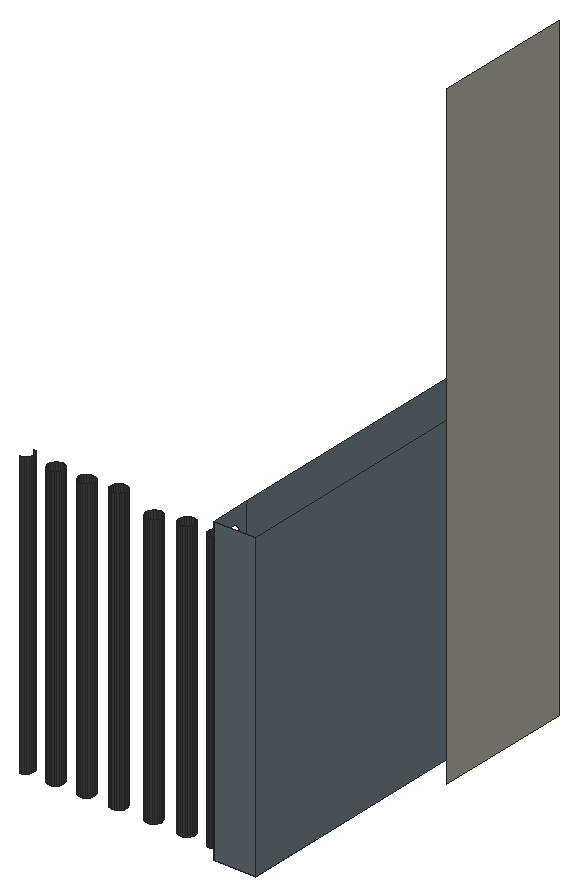
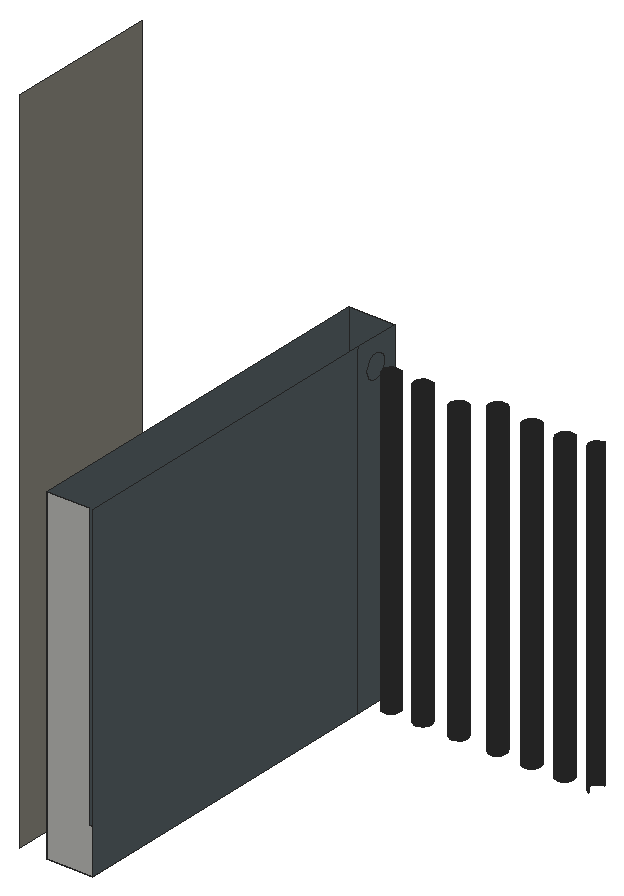
# SketchUp Ruby script. Lengths in inches.
U = 1.inch
M = Sketchup.active_model
def pt(a) = Geom::Point3d.new(a.map { |v| v * U })
def face(e, loops, mat)
  f = e.add_face(loops[0].map { |a| pt(a) })
  loops[1..].each { |l| e.add_face(l.map { |a| pt(a) }).erase! }
  f.material = f.back_material = mat if mat
  f
end
# faces: each face lists its corners as indices into pts; further lists are holes
def faces(e, pts, list, mat = nil) = list.each { |f| face(e, (f[0].is_a?(Array) ? f : [f]).map { |l| l.map { |i| pts[i] } }, mat) }
# xy, xz, yz: faces in a plane at the given z, y or x. An outline is a flat list of corners, or four numbers for a rectangle; further outlines are holes
def ring(l) = l.size == 4 ? [[l[0], l[1]], [l[2], l[1]], [l[2], l[3]], [l[0], l[3]]] : l.each_slice(2).to_a
def flat(e, list, mat, &to3) = list.each { |f| face(e, (f[0].is_a?(Array) ? f : [f]).map { |l| ring(l).map { |u, v| to3.(u, v) } }, mat) }
def xy(e, z, list, mat = nil) = flat(e, list, mat) { |x, y| [x, y, z] }
def xz(e, y, list, mat = nil) = flat(e, list, mat) { |x, z| [x, y, z] }
def yz(e, x, list, mat = nil) = flat(e, list, mat) { |y, z| [x, y, z] }
def lines(e, pts, list) = list.each { |a, b| e.add_line(pt(pts[a]), pt(pts[b])) }
# prism: a flat outline (further loops are holes) pulled along v
def prism(e, loops, v, mat = nil)
  f = face(e, loops, mat); d = Geom::Vector3d.new(v.map { |x| x * U })
  f.pushpull(f.normal.samedirection?(d) ? d.length : -d.length)
end
def box(e, o, s, mat = nil) = prism(e, [[o, [o[0] + s[0], o[1], o[2]], [o[0] + s[0], o[1] + s[1], o[2]], [o[0], o[1] + s[1], o[2]]]], [0, 0, s[2]], mat)
def at(x, y, z, deg = 0) = Geom::Transformation.translation(pt([x, y, z])) * Geom::Transformation.rotation(ORIGIN, Z_AXIS, deg.degrees)
def axes(o, x, y, z) = Geom::Transformation.new([*x, 0, *y, 0, *z, 0, *pt(o).to_a, 1])
def part(name) = M.definitions.add(name)
# library, detail: a bought-in or finely detailed component or shape, given as its bounding box
def library(name, o, s) = part(name).tap { |d| box(d.entities, o, s) }
def detail(e, o, s) = box(e.add_group.entities, o, s)
def put(e, d, t, mat = nil) = e.add_instance(d, t).tap { |i| i.material = mat if mat }
def group(e, t, mat = nil) = e.add_group.tap { |g| g.transformation = t; g.material = mat if mat }.entities
root = M.entities
M.materials.add("[Color M07]").color = [58, 58, 58]
M.materials.add("[Formica Graystone]").color = [149, 146, 135]
M.materials.add("[Formica Speckled Grey]").color = [94, 105, 111]
xy(root,557.29,[[289.43,116.47,292.74,144.04],[275.6,117.55,275.4375,117.57,275.29,117.63,275.16,117.73,275.06,117.86,275,118.01,274.98,118.17,275,118.33,275.06,118.48,275.16,118.61,275.29,118.71,275.4375,118.77,275.6,118.8,275.76,118.77,275.91,118.71,276.04,118.61,276.14,118.48,276.2,118.33,276.23,118.17,276.2,118.01,276.14,117.86,276.04,117.73,275.91,117.63,275.76,117.57],[278.04,117.55,277.875,117.57,277.73,117.63,277.6,117.73,277.5,117.86,277.43,118.01,277.41,118.17,277.43,118.33,277.5,118.48,277.6,118.61,277.73,118.71,277.875,118.77,278.04,118.8,278.2,118.77,278.35,118.71,278.48,118.61,278.58,118.48,278.64,118.33,278.66,118.17,278.64,118.01,278.58,117.86,278.48,117.73,278.35,117.63,278.2,117.57],[280.54,117.55,280.375,117.57,280.23,117.63,280.1,117.73,280,117.86,279.93,118.01,279.91,118.17,279.93,118.33,280,118.48,280.1,118.61,280.23,118.71,280.375,118.77,280.54,118.8,280.7,118.77,280.85,118.71,280.98,118.61,281.08,118.48,281.14,118.33,281.16,118.17,281.14,118.01,281.08,117.86,280.98,117.73,280.85,117.63,280.7,117.57],[283.35,117.55,283.1875,117.57,283.04,117.63,282.91,117.73,282.81,117.86,282.75,118.01,282.73,118.17,282.75,118.33,282.81,118.48,282.91,118.61,283.04,118.71,283.1875,118.77,283.35,118.8,283.51,118.77,283.66,118.71,283.79,118.61,283.89,118.48,283.95,118.33,283.98,118.17,283.95,118.01,283.89,117.86,283.79,117.73,283.66,117.63,283.51,117.57],
  [285.98,117.55,285.8125,117.57,285.66,117.63,285.53,117.73,285.43,117.86,285.37,118.01,285.35,118.17,285.37,118.33,285.43,118.48,285.53,118.61,285.66,118.71,285.8125,118.77,285.98,118.8,286.14,118.77,286.29,118.71,286.42,118.61,286.52,118.48,286.58,118.33,286.6,118.17,286.58,118.01,286.52,117.86,286.42,117.73,286.29,117.63,286.14,117.57],[288.29,117.55,288.125,117.57,287.98,117.63,287.85,117.73,287.75,117.86,287.68,118.01,287.66,118.17,287.68,118.33,287.75,118.48,287.85,118.61,287.98,118.71,288.125,118.77,288.29,118.8,288.45,118.77,288.6,118.71,288.73,118.61,288.83,118.48,288.89,118.33,288.91,118.17,288.89,118.01,288.83,117.86,288.73,117.73,288.6,117.63,288.45,117.57]])
xz(root,116.47,[[289.43,557.29,292.74,581.29]],"[Formica Speckled Grey]")
xz(root,144.04,[[289.43,557.29,292.74,557.29,292.74,581.29,289.71,581.29,289.71,560.54,289.43,560.54]])
yz(root,289.43,[[[116.47,557.29,119.78,581.29],[118.19,578.44,118.41,578.47,118.62,578.56,118.8,578.7,118.94,578.88,119.03,579.09,119.06,579.32,119.03,579.54,118.94,579.76,118.8,579.9375,118.62,580.08,118.41,580.16,118.19,580.19,117.96,580.16,117.75,580.08,117.57,579.9375,117.43,579.76,117.34,579.54,117.31,579.32,117.34,579.09,117.43,578.88,117.57,578.7,117.75,578.56,117.96,578.47]],[119.78,557.29,144.04,581.29]],"[Formica Speckled Grey]")
yz(root,292.74,[[116.47,557.29,144.04,581.29]],"[Formica Speckled Grey]")
yz(root,294.7,[[132.97,557.29,144.04,606.58]],"[Formica Graystone]")
p = [[273.23,117.55,557.29],[273.39,117.57,557.29],[273.39,117.57,578.7],[273.39,117.57,579.76],[273.23,117.55,579.76],[275.4375,117.57,557.29],
  [275.6,117.55,557.29],[275.6,117.55,579.54],[275.4375,117.57,579.54],[275.4375,117.57,578.7],[275.76,117.57,557.29],[275.76,117.57,578.7],
  [275.76,117.57,579.54],[277.875,117.57,557.29],[278.04,117.55,557.29],[278.04,117.55,579.54],[277.875,117.57,579.54],[277.875,117.57,578.7],
  [278.2,117.57,557.29],[278.2,117.57,578.7],[278.2,117.57,579.54],[280.375,117.57,557.29],[280.54,117.55,557.29],[280.54,117.55,579.76],
  [280.375,117.57,579.76],[280.375,117.57,578.7],[280.7,117.57,557.29],[280.7,117.57,578.7],[280.7,117.57,579.76],[283.1875,117.57,557.29],
  [283.35,117.55,557.29],[283.35,117.55,578.86],[283.1875,117.57,578.86],[283.1875,117.57,578.7],[283.51,117.57,557.29],[283.51,117.57,578.7],
  [283.51,117.57,578.86],[285.8125,117.57,557.29],[285.98,117.55,557.29],[285.98,117.55,579.32],[285.8125,117.57,579.32],[285.8125,117.57,578.7],
  [286.14,117.57,557.29],[286.14,117.57,578.7],[286.14,117.57,579.32],[288.125,117.57,557.29],[288.29,117.55,557.29],[288.29,117.55,579.29],
  [288.125,117.57,579.29],[288.125,117.57,578.7],[288.45,117.57,557.29],[288.45,117.57,578.7],[288.45,117.57,579.29],[273.54,117.63,557.29],
  [273.54,117.63,579.76],[273.67,117.73,557.29],[273.67,117.73,579.76],[275.16,117.73,557.29],[275.29,117.63,557.29],[275.29,117.63,579.54],
  [275.16,117.73,579.54],[275.91,117.63,557.29],[275.91,117.63,579.54],[276.04,117.73,557.29],[276.04,117.73,579.54],[277.6,117.73,557.29],
  [277.73,117.63,557.29],[277.73,117.63,579.54],[277.6,117.73,579.54],[278.35,117.63,557.29],[278.35,117.63,579.54],[278.48,117.73,557.29],
  [278.48,117.73,579.54],[280.1,117.73,557.29],[280.23,117.63,557.29],[280.23,117.63,579.76],[280.1,117.73,579.76],[280.85,117.63,557.29],
  [280.85,117.63,579.76],[280.98,117.73,557.29],[280.98,117.73,579.76],[282.91,117.73,557.29],[283.04,117.63,557.29],[283.04,117.63,578.86],
  [282.91,117.73,578.86],[283.66,117.63,557.29],[283.66,117.63,578.86],[283.79,117.73,557.29],[283.79,117.73,578.86],[285.53,117.73,557.29],
  [285.66,117.63,557.29],[285.66,117.63,579.32],[285.53,117.73,579.32],[286.29,117.63,557.29],[286.29,117.63,579.32],[286.42,117.73,557.29],
  [286.42,117.73,579.32],[287.85,117.73,557.29],[287.98,117.63,557.29],[287.98,117.63,579.29],[287.85,117.73,579.29],[288.6,117.63,557.29],
  [288.6,117.63,579.29],[288.73,117.73,557.29],[288.73,117.73,579.29],[273.77,117.86,557.29],[273.77,117.86,579.76],[275.06,117.86,557.29],
  [275.06,117.86,579.54],[276.14,117.86,557.29],[276.14,117.86,579.54],[277.5,117.86,557.29],[277.5,117.86,579.54],[278.58,117.86,557.29],
  [278.58,117.86,579.54],[280,117.86,557.29],[280,117.86,579.76],[281.08,117.86,557.29],[281.08,117.86,579.76],[282.81,117.86,557.29],
  [282.81,117.86,578.86],[283.89,117.86,557.29],[283.89,117.86,578.86],[285.43,117.86,557.29],[285.43,117.86,579.32],[286.52,117.86,557.29],
  [286.52,117.86,579.32],[287.75,117.86,557.29],[287.75,117.86,579.29],[288.83,117.86,557.29],[288.83,117.86,579.29],[273.83,118.01,557.29],
  [273.83,118.01,579.76],[275,118.01,557.29],[275,118.01,579.54],[276.2,118.01,557.29],[276.2,118.01,579.54],[277.43,118.01,557.29],
  [277.43,118.01,579.54],[278.64,118.01,557.29],[278.64,118.01,579.54],[279.93,118.01,557.29],[279.93,118.01,579.76],[281.14,118.01,557.29],
  [281.14,118.01,579.76],[282.75,118.01,557.29],[282.75,118.01,578.86],[283.95,118.01,557.29],[283.95,118.01,578.86],[285.37,118.01,557.29],
  [285.37,118.01,579.32],[286.58,118.01,557.29],[286.58,118.01,579.32],[287.68,118.01,557.29],[287.68,118.01,579.29],[288.89,118.01,557.29],
  [288.89,118.01,579.29],[273.85,118.17,557.29],[273.85,118.17,579.76],[274.98,118.17,557.29],[274.98,118.17,579.54],[276.23,118.17,557.29],
  [276.23,118.17,579.54],[277.41,118.17,557.29],[277.41,118.17,579.54],[278.66,118.17,557.29],[278.66,118.17,579.54],[279.91,118.17,557.29],
  [279.91,118.17,579.76],[281.16,118.17,557.29],[281.16,118.17,579.76],[282.73,118.17,557.29],[282.73,118.17,578.86],[283.98,118.17,557.29],
  [283.98,118.17,578.86],[285.35,118.17,557.29],[285.35,118.17,579.32],[286.6,118.17,557.29],[286.6,118.17,579.32],[287.66,118.17,557.29],
  [287.66,118.17,579.29],[288.91,118.17,557.29],[288.91,118.17,579.29],[273.83,118.33,557.29],[273.83,118.33,579.76],[275,118.33,557.29],
  [275,118.33,579.54],[276.2,118.33,557.29],[276.2,118.33,579.54],[277.43,118.33,557.29],[277.43,118.33,579.54],[278.64,118.33,557.29],
  [278.64,118.33,579.54],[279.93,118.33,557.29],[279.93,118.33,579.76],[281.14,118.33,557.29],[281.14,118.33,579.76],[282.75,118.33,557.29],
  [282.75,118.33,578.86],[283.95,118.33,557.29],[283.95,118.33,578.86],[285.37,118.33,557.29],[285.37,118.33,579.32],[286.58,118.33,557.29],
  [286.58,118.33,579.32],[287.68,118.33,557.29],[287.68,118.33,579.29],[288.89,118.33,557.29],[288.89,118.33,579.29],[273.77,118.48,557.29],
  [273.77,118.48,579.76],[275.06,118.48,557.29],[275.06,118.48,579.54],[276.14,118.48,557.29],[276.14,118.48,579.54],[277.5,118.48,557.29],
  [277.5,118.48,579.54],[278.58,118.48,557.29],[278.58,118.48,579.54],[280,118.48,557.29],[280,118.48,579.76],[281.08,118.48,557.29],
  [281.08,118.48,579.76],[282.81,118.48,557.29],[282.81,118.48,578.86],[283.89,118.48,557.29],[283.89,118.48,578.86],[285.43,118.48,557.29],
  [285.43,118.48,579.32],[286.52,118.48,557.29],[286.52,118.48,579.32],[287.75,118.48,557.29],[287.75,118.48,579.29],[288.83,118.48,557.29],
  [288.83,118.48,579.29],[273.67,118.61,557.29],[273.67,118.61,579.76],[275.16,118.61,557.29],[275.16,118.61,579.54],[276.04,118.61,557.29],
  [276.04,118.61,579.54],[277.6,118.61,557.29],[277.6,118.61,579.54],[278.48,118.61,557.29],[278.48,118.61,579.54],[280.1,118.61,557.29],
  [280.1,118.61,579.76],[280.98,118.61,557.29],[280.98,118.61,579.76],[282.91,118.61,557.29],[282.91,118.61,578.86],[283.79,118.61,557.29],
  [283.79,118.61,578.86],[285.53,118.61,557.29],[285.53,118.61,579.32],[286.42,118.61,557.29],[286.42,118.61,579.32],[287.85,118.61,557.29],
  [287.85,118.61,579.29],[288.73,118.61,557.29],[288.73,118.61,579.29],[273.54,118.71,557.29],[273.54,118.71,579.76],[275.29,118.71,557.29],
  [275.29,118.71,579.54],[275.91,118.71,557.29],[275.91,118.71,579.54],[277.73,118.71,557.29],[277.73,118.71,579.54],[278.35,118.71,557.29],
  [278.35,118.71,579.54],[280.23,118.71,557.29],[280.23,118.71,579.76],[280.85,118.71,557.29],[280.85,118.71,579.76],[283.04,118.71,557.29],
  [283.04,118.71,578.86],[283.66,118.71,557.29],[283.66,118.71,578.86],[285.66,118.71,557.29],[285.66,118.71,579.32],[286.29,118.71,557.29],
  [286.29,118.71,579.32],[287.98,118.71,557.29],[287.98,118.71,579.29],[288.6,118.71,557.29],[288.6,118.71,579.29],[273.39,118.77,557.29],
  [273.39,118.77,579.76],[275.4375,118.77,557.29],[275.4375,118.77,579.54],[275.76,118.77,557.29],[275.76,118.77,579.54],[277.875,118.77,557.29],
  [277.875,118.77,579.54],[278.2,118.77,557.29],[278.2,118.77,579.54],[280.375,118.77,557.29],[280.375,118.77,579.76],[280.7,118.77,557.29],
  [280.7,118.77,579.76],[283.1875,118.77,557.29],[283.1875,118.77,578.86],[283.51,118.77,557.29],[283.51,118.77,578.86],[285.8125,118.77,557.29],
  [285.8125,118.77,579.32],[286.14,118.77,557.29],[286.14,118.77,579.32],[288.125,118.77,557.29],[288.125,118.77,579.29],[288.45,118.77,557.29],
  [288.45,118.77,579.29],[275.6,118.8,557.29],[275.6,118.8,579.54],[278.04,118.8,557.29],[278.04,118.8,579.54],[280.54,118.8,557.29],
  [280.54,118.8,579.76],[283.35,118.8,557.29],[283.35,118.8,578.86],[285.98,118.8,557.29],[285.98,118.8,579.32],[288.29,118.8,557.29],
  [288.29,118.8,579.29]]
faces(root,p,[[0,1,2,3,4],[5,6,7,8,9],[6,10,11,12,7],[13,14,15,16,17],[14,18,19,20,15],[21,22,23,24,25],[22,26,27,28,23],[29,30,31,32,33],
  [30,34,35,36,31],[37,38,39,40,41],[38,42,43,44,39],[45,46,47,48,49],[46,50,51,52,47],[1,53,54,3,2],[53,55,56,54],[57,58,59,60],
  [58,5,9,8,59],[10,61,62,12,11],[61,63,64,62],[65,66,67,68],[66,13,17,16,67],[18,69,70,20,19],[69,71,72,70],[73,74,75,76],
  [74,21,25,24,75],[26,77,78,28,27],[77,79,80,78],[81,82,83,84],[82,29,33,32,83],[34,85,86,36,35],[85,87,88,86],[89,90,91,92],
  [90,37,41,40,91],[42,93,94,44,43],[93,95,96,94],[97,98,99,100],[98,45,49,48,99],[50,101,102,52,51],[101,103,104,102],[55,105,106,56],
  [107,57,60,108],[63,109,110,64],[111,65,68,112],[71,113,114,72],[115,73,76,116],[79,117,118,80],[119,81,84,120],[87,121,122,88],
  [123,89,92,124],[95,125,126,96],[127,97,100,128],[103,129,130,104],[105,131,132,106],[133,107,108,134],[109,135,136,110],[137,111,112,138],
  [113,139,140,114],[141,115,116,142],[117,143,144,118],[145,119,120,146],[121,147,148,122],[149,123,124,150],[125,151,152,126],[153,127,128,154],
  [129,155,156,130],[131,157,158,132],[159,133,134,160],[135,161,162,136],[163,137,138,164],[139,165,166,140],[167,141,142,168],[143,169,170,144],
  [171,145,146,172],[147,173,174,148],[175,149,150,176],[151,177,178,152],[179,153,154,180],[155,181,182,156],[157,183,184,158],[185,159,160,186],
  [161,187,188,162],[189,163,164,190],[165,191,192,166],[193,167,168,194],[169,195,196,170],[197,171,172,198],[173,199,200,174],[201,175,176,202],
  [177,203,204,178],[205,179,180,206],[181,207,208,182],[183,209,210,184],[211,185,186,212],[187,213,214,188],[215,189,190,216],[191,217,218,192],
  [219,193,194,220],[195,221,222,196],[223,197,198,224],[199,225,226,200],[227,201,202,228],[203,229,230,204],[231,205,206,232],[207,233,234,208],
  [209,235,236,210],[237,211,212,238],[213,239,240,214],[241,215,216,242],[217,243,244,218],[245,219,220,246],[221,247,248,222],[249,223,224,250],
  [225,251,252,226],[253,227,228,254],[229,255,256,230],[257,231,232,258],[233,259,260,234],[235,261,262,236],[263,237,238,264],[239,265,266,240],
  [267,241,242,268],[243,269,270,244],[271,245,246,272],[247,273,274,248],[275,249,250,276],[251,277,278,252],[279,253,254,280],[255,281,282,256],
  [283,257,258,284],[259,285,286,260],[261,287,288,262],[289,263,264,290],[265,291,292,266],[293,267,268,294],[269,295,296,270],[297,271,272,298],
  [273,299,300,274],[301,275,276,302],[277,303,304,278],[305,279,280,306],[281,307,308,282],[309,283,284,310],[285,311,312,286],[313,289,290,314],
  [291,313,314,292],[315,293,294,316],[295,315,316,296],[317,297,298,318],[299,317,318,300],[319,301,302,320],[303,319,320,304],[321,305,306,322],
  [307,321,322,308],[323,309,310,324],[311,323,324,312]],"[Color M07]")
